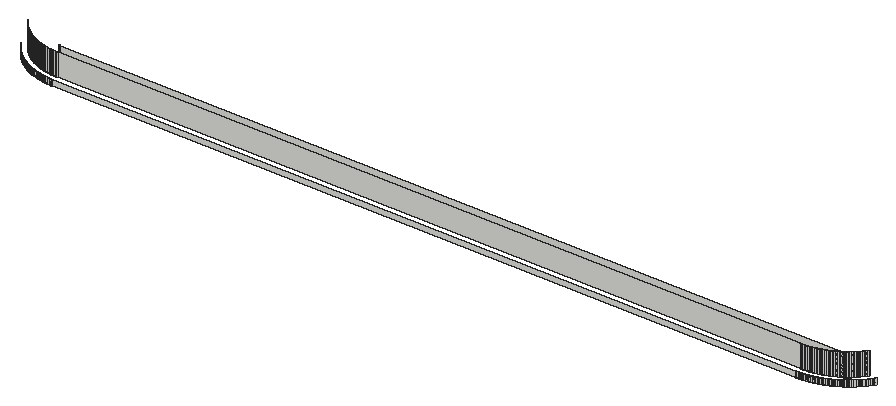
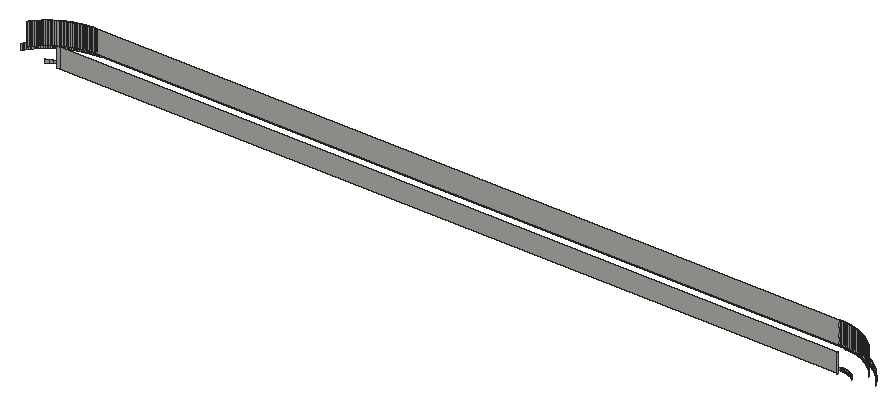
# SketchUp Ruby script. Lengths in inches.
U = 1.inch
M = Sketchup.active_model
def pt(a) = Geom::Point3d.new(a.map { |v| v * U })
def face(e, loops, mat)
  f = e.add_face(loops[0].map { |a| pt(a) })
  loops[1..].each { |l| e.add_face(l.map { |a| pt(a) }).erase! }
  f.material = f.back_material = mat if mat
  f
end
# faces: each face lists its corners as indices into pts; further lists are holes
def faces(e, pts, list, mat = nil) = list.each { |f| face(e, (f[0].is_a?(Array) ? f : [f]).map { |l| l.map { |i| pts[i] } }, mat) }
# xy, xz, yz: faces in a plane at the given z, y or x. An outline is a flat list of corners, or four numbers for a rectangle; further outlines are holes
def ring(l) = l.size == 4 ? [[l[0], l[1]], [l[2], l[1]], [l[2], l[3]], [l[0], l[3]]] : l.each_slice(2).to_a
def flat(e, list, mat, &to3) = list.each { |f| face(e, (f[0].is_a?(Array) ? f : [f]).map { |l| ring(l).map { |u, v| to3.(u, v) } }, mat) }
def xy(e, z, list, mat = nil) = flat(e, list, mat) { |x, y| [x, y, z] }
def xz(e, y, list, mat = nil) = flat(e, list, mat) { |x, z| [x, y, z] }
def yz(e, x, list, mat = nil) = flat(e, list, mat) { |y, z| [x, y, z] }
def lines(e, pts, list) = list.each { |a, b| e.add_line(pt(pts[a]), pt(pts[b])) }
# prism: a flat outline (further loops are holes) pulled along v
def prism(e, loops, v, mat = nil)
  f = face(e, loops, mat); d = Geom::Vector3d.new(v.map { |x| x * U })
  f.pushpull(f.normal.samedirection?(d) ? d.length : -d.length)
end
def box(e, o, s, mat = nil) = prism(e, [[o, [o[0] + s[0], o[1], o[2]], [o[0] + s[0], o[1] + s[1], o[2]], [o[0], o[1] + s[1], o[2]]]], [0, 0, s[2]], mat)
def at(x, y, z, deg = 0) = Geom::Transformation.translation(pt([x, y, z])) * Geom::Transformation.rotation(ORIGIN, Z_AXIS, deg.degrees)
def axes(o, x, y, z) = Geom::Transformation.new([*x, 0, *y, 0, *z, 0, *pt(o).to_a, 1])
def part(name) = M.definitions.add(name)
# library, detail: a bought-in or finely detailed component or shape, given as its bounding box
def library(name, o, s) = part(name).tap { |d| box(d.entities, o, s) }
def detail(e, o, s) = box(e.add_group.entities, o, s)
def put(e, d, t, mat = nil) = e.add_instance(d, t).tap { |i| i.material = mat if mat }
def group(e, t, mat = nil) = e.add_group.tap { |g| g.transformation = t; g.material = mat if mat }.entities
root = M.entities
xz(root,144,[[23.87,120,24.1875,122],[24.1875,120,290.26,122],[290.26,120,290.58,122]])
xz(root,146,[[23.9,122,24.1875,130],[24.1875,122,290.26,130],[290.26,122,290.55,130]])
xz(root,153,[[17.82,119,18,120],[18,119,296.45,120]])
xz(root,155,[[17.86,119,18,126],[18,119,296.45,126]])
xz(root,155.01,[[17.59,119,17.73,126]])
p = [[17.12,153.04,120],[16.94,153.0625,120],[16.94,153.0625,119],[17.12,153.04,119],[17.29,153.03,120],[17.29,153.03,119],
  [17.47,153.02,120],[17.47,153.02,119],[17.65,153.01,120],[17.65,153.01,119],[17.82,153,120],[17.82,153,119],
  [297.63,153.08,120],[296.45,153,120],[296.45,153,119],[297.63,153.08,119],[16.42,153.14,120],[16.24,153.17,120],
  [16.24,153.17,119],[16.42,153.14,119],[16.59,153.11,120],[16.59,153.11,119],[16.77,153.08,120],[16.77,153.08,119],
  [298.78,153.31,120],[298.78,153.31,119],[15.9,153.25,120],[15.73,153.29,120],[15.73,153.29,119],[15.9,153.25,119],
  [16.07,153.21,120],[16.07,153.21,119],[15.56,153.34,120],[15.39,153.39,120],[15.39,153.39,119],[15.56,153.34,119],
  [299.9,153.69,120],[299.9,153.69,119],[15.22,153.44,120],[15.05,153.5,120],[15.05,153.5,119],[15.22,153.44,119],
  [14.88,153.56,120],[14.88,153.56,119],[14.72,153.62,120],[14.56,153.69,120],[14.56,153.69,119],[14.72,153.62,119],
  [14.39,153.75,120],[14.39,153.75,119],[300.95,154.21,120],[300.95,154.21,119],[14.23,153.83,120],[14.07,153.9,120],
  [14.07,153.9,119],[14.23,153.83,119],[13.91,153.98,120],[13.91,153.98,119],[13.76,154.0625,120],[13.76,154.0625,119],
  [13.6,154.15,120],[13.45,154.24,120],[13.45,154.24,119],[13.6,154.15,119],[13.3,154.33,120],[13.3,154.33,119],
  [301.93,154.86,120],[301.93,154.86,119],[13.15,154.42,120],[13.15,154.42,119],[13,154.52,120],[13,154.52,119],
  [12.85,154.62,120],[12.85,154.62,119],[12.71,154.72,120],[12.71,154.72,119],[12.57,154.82,120],[12.57,154.82,119],
  [12.43,154.93,120],[12.43,154.93,119],[12.29,155.04,120],[12.29,155.04,119],[17.3125,155.03,126],[17.45,155.02,126],
  [17.45,155.02,119],[17.3125,155.03,119],[17.59,155.01,126],[17.59,155.01,119],[17.73,155.01,126],[17.86,155,126],
  [17.86,155,119],[17.73,155.01,119],[296.45,155,126],[297.37,155.06,126],[297.37,155.06,119],[296.45,155,119],
  [22.61,144.05,120],[22.92,144.03,120],[22.92,144.03,122],[22.61,144.05,122],[23.24,144.02,120],[23.24,144.02,122],
  [23.56,144.01,120],[23.56,144.01,122],[23.87,144,120],[23.87,144,122],[290.58,144,120],[290.9,144.01,120],
  [290.9,144.01,122],[290.58,144,122],[291.21,144.02,120],[291.21,144.02,122],[291.53,144.03,120],[291.53,144.03,122],
  [291.85,144.05,120],[291.85,144.05,122],[21.35,144.17,120],[21.66,144.13,120],[21.66,144.13,122],[21.35,144.17,122],
  [21.98,144.1,120],[21.98,144.1,122],[22.29,144.07,120],[22.29,144.07,122],[292.16,144.07,120],[292.16,144.07,122],
  [292.48,144.1,120],[292.48,144.1,122],[292.79,144.13,120],[292.79,144.13,122],[293.11,144.17,120],[293.11,144.17,122],
  [20.4,144.3,120],[20.72,144.25,120],[20.72,144.25,122],[20.4,144.3,122],[21.03,144.21,120],[21.03,144.21,122],
  [293.42,144.21,120],[293.42,144.21,122],[293.74,144.25,120],[293.74,144.25,122],[294.05,144.3,120],[294.05,144.3,122],
  [19.78,144.4,120],[20.09,144.35,120],[20.09,144.35,122],[19.78,144.4,122],[294.36,144.35,120],[294.36,144.35,122],
  [294.67,144.4,120],[294.67,144.4,122],[19.47,144.46,120],[19.47,144.46,122],[294.98,144.46,120],[294.98,144.46,122],
  [18.85,144.59,120],[19.16,144.52,120],[19.16,144.52,122],[18.85,144.59,122],[295.29,144.52,120],[295.29,144.52,122],
  [295.6,144.59,120],[295.6,144.59,122],[18.54,144.66,120],[18.54,144.66,122],[295.91,144.66,120],[295.91,144.66,122],
  [17.93,144.82,120],[18.23,144.74,120],[18.23,144.74,122],[17.93,144.82,122],[296.22,144.74,120],[296.22,144.74,122],
  [296.53,144.82,120],[296.53,144.82,122],[17.62,144.9,120],[17.62,144.9,122],[296.83,144.9,120],[296.83,144.9,122],
  [17.32,144.99,120],[17.32,144.99,122],[297.13,144.99,120],[297.13,144.99,122],[17.02,145.08,120],[17.02,145.08,122],
  [297.4375,145.08,120],[297.4375,145.08,122],[16.71,145.17,120],[16.71,145.17,122],[297.74,145.17,120],[297.74,145.17,122],
  [16.41,145.27,120],[16.41,145.27,122],[298.04,145.27,120],[298.04,145.27,122],[16.11,145.375,120],[16.11,145.375,122],
  [298.34,145.375,120],[298.34,145.375,122],[15.82,145.48,120],[15.82,145.48,122],[298.64,145.48,120],[298.64,145.48,122],
  [15.52,145.59,120],[15.52,145.59,122],[298.93,145.59,120],[298.93,145.59,122],[15.23,145.71,120],[15.23,145.71,122],
  [299.23,145.71,120],[299.23,145.71,122],[14.93,145.83,120],[14.93,145.83,122],[299.52,145.83,120],[299.52,145.83,122],
  [14.64,145.95,120],[14.64,145.95,122],[299.8125,145.95,120],[299.8125,145.95,122],[14.35,146.07,120],[14.35,146.07,122],
  [300.1,146.07,120],[300.1,146.07,122],[14.0625,146.2,120],[14.0625,146.2,122],[300.39,146.2,120],[300.39,146.2,122],
  [13.78,146.34,120],[13.78,146.34,122],[300.68,146.34,120],[300.68,146.34,122],[13.49,146.48,120],[13.49,146.48,122],
  [300.96,146.48,120],[300.96,146.48,122],[13.21,146.62,120],[13.21,146.62,122],[301.25,146.62,120],[301.25,146.62,122],
  [12.93,146.76,120],[12.93,146.76,122],[301.53,146.76,120],[301.53,146.76,122],[12.65,146.91,120],[12.65,146.91,122],
  [301.81,146.91,120],[301.81,146.91,122],[12.37,147.06,120],[12.37,147.06,122],[302.08,147.06,120],[302.08,147.06,122],
  [12.09,147.22,120],[12.09,147.22,122],[302.36,147.22,120],[302.36,147.22,122],[11.82,147.375,120],[11.82,147.375,122],
  [302.63,147.375,120],[302.63,147.375,122],[11.55,147.54,120],[11.55,147.54,122],[302.9,147.54,120],[302.9,147.54,122],
  [11.28,147.7,120],[11.28,147.7,122],[303.17,147.7,120],[303.17,147.7,122],[11.01,147.87,120],[11.01,147.87,122],
  [303.4375,147.87,120],[303.4375,147.87,122],[10.75,148.04,120],[10.75,148.04,122],[303.7,148.04,120],[303.7,148.04,122],
  [10.49,148.22,120],[10.49,148.22,122],[303.97,148.22,120],[303.97,148.22,122],[10.23,148.4,120],[10.23,148.4,122],
  [304.23,148.4,120],[304.23,148.4,122],[9.97,148.58,120],[9.97,148.58,122],[304.48,148.58,120],[304.48,148.58,122],
  [9.72,148.77,120],[9.72,148.77,122],[304.74,148.77,120],[304.74,148.77,122],[9.46,148.96,120],[9.46,148.96,122],
  [304.99,148.96,120],[304.99,148.96,122],[9.21,149.15,120],[9.21,149.15,122],[305.24,149.15,120],[305.24,149.15,122],
  [8.97,149.35,120],[8.97,149.35,122],[305.49,149.35,120],[305.49,149.35,122],[8.72,149.55,120],[8.72,149.55,122],
  [305.73,149.55,120],[305.73,149.55,122],[8.48,149.75,120],[8.48,149.75,122],[305.97,149.75,120],[305.97,149.75,122],
  [8.24,149.96,120],[8.24,149.96,122],[306.21,149.96,120],[306.21,149.96,122],[8,150.16,120],[8,150.16,122],
  [306.45,150.16,120],[306.45,150.16,122],[7.77,150.375,120],[7.77,150.375,122],[306.68,150.375,120],[306.68,150.375,122],
  [7.54,150.59,120],[7.54,150.59,122],[306.92,150.59,120],[306.92,150.59,122],[7.31,150.81,120],[7.31,150.81,122],
  [307.14,150.81,120],[307.14,150.81,122],[7.08,151.03,120],[7.08,151.03,122],[307.37,151.03,120],[307.37,151.03,122],
  [6.86,151.25,120],[6.86,151.25,122],[307.59,151.25,120],[307.59,151.25,122],[6.64,151.48,120],[6.64,151.48,122],
  [307.8125,151.48,120],[307.8125,151.48,122],[6.43,151.71,120],[6.43,151.71,122],[308.03,151.71,120],[308.03,151.71,122],
  [6.21,151.94,120],[6.21,151.94,122],[308.24,151.94,120],[308.24,151.94,122],[6,152.18,120],[6,152.18,122],
  [308.45,152.18,120],[308.45,152.18,122],[5.8,152.41,120],[5.8,152.41,122],[308.66,152.41,120],[308.66,152.41,122],
  [5.59,152.65,120],[5.59,152.65,122],[308.86,152.65,120],[308.86,152.65,122],[5.39,152.9,120],[5.39,152.9,122],
  [309.0625,152.9,120],[309.0625,152.9,122],[5.19,153.14,120],[5.19,153.14,122],[309.26,153.14,120],[309.26,153.14,122],
  [5,153.39,120],[5,153.39,122],[309.45,153.39,120],[309.45,153.39,122],[4.81,153.64,120],[4.81,153.64,122],
  [309.65,153.64,120],[309.65,153.64,122],[4.62,153.89,120],[4.62,153.89,122],[309.83,153.89,120],[309.83,153.89,122],
  [4.44,154.15,120],[4.44,154.15,122],[310.02,154.15,120],[310.02,154.15,122],[4.25,154.41,120],[4.25,154.41,122],
  [310.2,154.41,120],[310.2,154.41,122],[4.08,154.67,120],[4.08,154.67,122],[310.375,154.67,120],[310.375,154.67,122],
  [3.9,154.93,120],[3.9,154.93,122],[310.55,154.93,120],[310.55,154.93,122],[22.45,146.07,122],[22.74,146.05,122],
  [22.74,146.05,130],[22.45,146.07,130],[23.03,146.03,122],[23.03,146.03,130],[23.32,146.02,122],[23.32,146.02,130],
  [23.61,146.01,122],[23.61,146.01,130],[23.9,146,122],[23.9,146,130],[290.55,146,122],[290.85,146.01,122],
  [290.85,146.01,130],[290.55,146,130],[291.14,146.02,122],[291.14,146.02,130],[291.43,146.03,122],[291.43,146.03,130],
  [291.71,146.05,122],[291.71,146.05,130],[292,146.07,122],[292,146.07,130],[21.58,146.15,122],[21.87,146.12,122],
  [21.87,146.12,130],[21.58,146.15,130],[22.16,146.09,122],[22.16,146.09,130],[292.29,146.09,122],[292.29,146.09,130],
  [292.58,146.12,122],[292.58,146.12,130],[292.87,146.15,122],[292.87,146.15,130],[20.72,146.27,122],[21.01,146.23,122],
  [21.01,146.23,130],[20.72,146.27,130],[21.29,146.1875,122],[21.29,146.1875,130],[293.16,146.1875,122],[293.16,146.1875,130],
  [293.45,146.23,122],[293.45,146.23,130],[293.73,146.27,122],[293.73,146.27,130],[20.15,146.37,122],[20.43,146.32,122],
  [20.43,146.32,130],[20.15,146.37,130],[294.02,146.32,122],[294.02,146.32,130],[294.31,146.37,122],[294.31,146.37,130],
  [19.58,146.48,122],[19.86,146.42,122],[19.86,146.42,130],[19.58,146.48,130],[294.59,146.42,122],[294.59,146.42,130],
  [294.875,146.48,122],[294.875,146.48,130],[19.01,146.61,122],[19.3,146.54,122],[19.3,146.54,130],[19.01,146.61,130],
  [295.16,146.54,122],[295.16,146.54,130],[295.44,146.61,122],[295.44,146.61,130],[18.73,146.68,122],[18.73,146.68,130],
  [295.72,146.68,122],[295.72,146.68,130],[18.17,146.83,122],[18.45,146.75,122],[18.45,146.75,130],[18.17,146.83,130],
  [296,146.75,122],[296,146.75,130],[296.28,146.83,122],[296.28,146.83,130],[17.89,146.91,122],[17.89,146.91,130],
  [296.5625,146.91,122],[296.5625,146.91,130],[17.61,146.99,122],[17.61,146.99,130],[296.84,146.99,122],[296.84,146.99,130],
  [17.34,147.08,122],[17.34,147.08,130],[297.12,147.08,122],[297.12,147.08,130],[17.0625,147.17,122],[17.0625,147.17,130],
  [297.39,147.17,122],[297.39,147.17,130],[16.79,147.26,122],[16.79,147.26,130],[297.67,147.26,122],[297.67,147.26,130],
  [16.51,147.36,122],[16.51,147.36,130],[297.9375,147.36,122],[297.9375,147.36,130],[16.24,147.46,122],[16.24,147.46,130],
  [298.21,147.46,122],[298.21,147.46,130],[15.97,147.57,122],[15.97,147.57,130],[298.48,147.57,122],[298.48,147.57,130],
  [15.7,147.67,122],[15.7,147.67,130],[298.75,147.67,122],[298.75,147.67,130],[15.4375,147.79,122],[15.4375,147.79,130],
  [299.02,147.79,122],[299.02,147.79,130],[15.17,147.9,122],[15.17,147.9,130],[299.28,147.9,122],[299.28,147.9,130],
  [14.91,148.02,122],[14.91,148.02,130],[299.55,148.02,122],[299.55,148.02,130],[14.64,148.14,122],[14.64,148.14,130],
  [299.81,148.14,122],[299.81,148.14,130],[14.38,148.27,122],[14.38,148.27,130],[300.07,148.27,122],[300.07,148.27,130],
  [14.12,148.4,122],[14.12,148.4,130],[300.33,148.4,122],[300.33,148.4,130],[13.86,148.53,122],[13.86,148.53,130],
  [300.59,148.53,122],[300.59,148.53,130],[13.61,148.67,122],[13.61,148.67,130],[300.84,148.67,122],[300.84,148.67,130],
  [13.35,148.81,122],[13.35,148.81,130],[301.1,148.81,122],[301.1,148.81,130],[13.1,148.95,122],[13.1,148.95,130],
  [301.35,148.95,122],[301.35,148.95,130],[12.85,149.09,122],[12.85,149.09,130],[301.6,149.09,122],[301.6,149.09,130],
  [12.6,149.24,122],[12.6,149.24,130],[301.85,149.24,122],[301.85,149.24,130],[12.36,149.39,122],[12.36,149.39,130],
  [302.1,149.39,122],[302.1,149.39,130],[12.11,149.55,122],[12.11,149.55,130],[302.34,149.55,122],[302.34,149.55,130],
  [11.87,149.71,122],[11.87,149.71,130],[302.58,149.71,122],[302.58,149.71,130],[11.63,149.87,122],[11.63,149.87,130],
  [302.82,149.87,122],[302.82,149.87,130],[11.39,150.03,122],[11.39,150.03,130],[303.0625,150.03,122],[303.0625,150.03,130],
  [11.16,150.2,122],[11.16,150.2,130],[303.3,150.2,122],[303.3,150.2,130],[10.92,150.37,122],[10.92,150.37,130],
  [303.53,150.37,122],[303.53,150.37,130],[10.69,150.55,122],[10.69,150.55,130],[303.76,150.55,122],[303.76,150.55,130],
  [10.46,150.72,122],[10.46,150.72,130],[303.99,150.72,122],[303.99,150.72,130],[10.23,150.9,122],[10.23,150.9,130],
  [304.22,150.9,122],[304.22,150.9,130],[10.01,151.09,122],[10.01,151.09,130],[304.44,151.09,122],[304.44,151.09,130],
  [9.79,151.27,122],[9.79,151.27,130],[304.66,151.27,122],[304.66,151.27,130],[9.57,151.46,122],[9.57,151.46,130],
  [304.88,151.46,122],[304.88,151.46,130],[9.35,151.65,122],[9.35,151.65,130],[305.1,151.65,122],[305.1,151.65,130],
  [9.14,151.84,122],[9.14,151.84,130],[305.32,151.84,122],[305.32,151.84,130],[8.93,152.04,122],[8.93,152.04,130],
  [305.53,152.04,122],[305.53,152.04,130],[8.72,152.24,122],[8.72,152.24,130],[305.74,152.24,122],[305.74,152.24,130],
  [8.51,152.44,122],[8.51,152.44,130],[305.94,152.44,122],[305.94,152.44,130],[8.31,152.65,122],[8.31,152.65,130],
  [306.15,152.65,122],[306.15,152.65,130],[8.11,152.86,122],[8.11,152.86,130],[306.35,152.86,122],[306.35,152.86,130],
  [7.91,153.07,122],[7.91,153.07,130],[306.55,153.07,122],[306.55,153.07,130],[7.71,153.28,122],[7.71,153.28,130],
  [306.74,153.28,122],[306.74,153.28,130],[7.52,153.49,122],[7.52,153.49,130],[306.94,153.49,122],[306.94,153.49,130],
  [7.33,153.71,122],[7.33,153.71,130],[307.125,153.71,122],[307.125,153.71,130],[7.14,153.93,122],[7.14,153.93,130],
  [307.3125,153.93,122],[307.3125,153.93,130],[6.96,154.15,122],[6.96,154.15,130],[307.5,154.15,122],[307.5,154.15,130],
  [6.78,154.38,122],[6.78,154.38,130],[307.68,154.38,122],[307.68,154.38,130],[6.6,154.61,122],[6.6,154.61,130],
  [307.86,154.61,122],[307.86,154.61,130],[6.42,154.84,122],[6.42,154.84,130],[308.03,154.84,122],[308.03,154.84,130],
  [6.25,155.07,122],[6.25,155.07,130],[308.2,155.07,122],[308.2,155.07,130]]
faces(root,p,[[0,1,2,3],[4,0,3,5],[6,4,5,7],[8,6,7,9],[10,8,9,11],[12,13,14,15],[16,17,18,19],[20,16,19,21],
  [22,20,21,23],[1,22,23,2],[24,12,15,25],[26,27,28,29],[30,26,29,31],[17,30,31,18],[32,33,34,35],[27,32,35,28],
  [36,24,25,37],[38,39,40,41],[33,38,41,34],[39,42,43,40],[44,45,46,47],[42,44,47,43],[45,48,49,46],[50,36,37,51],
  [52,53,54,55],[48,52,55,49],[53,56,57,54],[56,58,59,57],[60,61,62,63],[58,60,63,59],[61,64,65,62],[66,50,51,67],
  [64,68,69,65],[68,70,71,69],[70,72,73,71],[72,74,75,73],[74,76,77,75],[76,78,79,77],[78,80,81,79],[82,83,84,85],
  [83,86,87,84],[88,89,90,91],[92,93,94,95],[96,97,98,99],[97,100,101,98],[100,102,103,101],[102,104,105,103],[106,107,108,109],
  [107,110,111,108],[110,112,113,111],[112,114,115,113],[116,117,118,119],[117,120,121,118],[120,122,123,121],[122,96,99,123],[114,124,125,115],
  [124,126,127,125],[126,128,129,127],[128,130,131,129],[132,133,134,135],[133,136,137,134],[136,116,119,137],[130,138,139,131],[138,140,141,139],
  [140,142,143,141],[144,145,146,147],[145,132,135,146],[142,148,149,143],[148,150,151,149],[152,144,147,153],[150,154,155,151],[156,157,158,159],
  [157,152,153,158],[154,160,161,155],[160,162,163,161],[164,156,159,165],[162,166,167,163],[168,169,170,171],[169,164,165,170],[166,172,173,167],
  [172,174,175,173],[176,168,171,177],[174,178,179,175],[180,176,177,181],[178,182,183,179],[184,180,181,185],[182,186,187,183],[188,184,185,189],
  [186,190,191,187],[192,188,189,193],[190,194,195,191],[196,192,193,197],[194,198,199,195],[200,196,197,201],[198,202,203,199],[204,200,201,205],
  [202,206,207,203],[208,204,205,209],[206,210,211,207],[212,208,209,213],[210,214,215,211],[216,212,213,217],[214,218,219,215],[220,216,217,221],
  [218,222,223,219],[224,220,221,225],[222,226,227,223],[228,224,225,229],[226,230,231,227],[232,228,229,233],[230,234,235,231],[236,232,233,237],
  [234,238,239,235],[240,236,237,241],[238,242,243,239],[244,240,241,245],[242,246,247,243],[248,244,245,249],[246,250,251,247],[252,248,249,253],
  [250,254,255,251],[256,252,253,257],[254,258,259,255],[260,256,257,261],[258,262,263,259],[264,260,261,265],[262,266,267,263],[268,264,265,269],
  [266,270,271,267],[272,268,269,273],[270,274,275,271],[276,272,273,277],[274,278,279,275],[280,276,277,281],[278,282,283,279],[284,280,281,285],
  [282,286,287,283],[288,284,285,289],[286,290,291,287],[292,288,289,293],[290,294,295,291],[296,292,293,297],[294,298,299,295],[300,296,297,301],
  [298,302,303,299],[304,300,301,305],[302,306,307,303],[308,304,305,309],[306,310,311,307],[312,308,309,313],[310,314,315,311],[316,312,313,317],
  [314,318,319,315],[320,316,317,321],[318,322,323,319],[324,320,321,325],[322,326,327,323],[328,324,325,329],[326,330,331,327],[332,328,329,333],
  [330,334,335,331],[336,332,333,337],[334,338,339,335],[340,336,337,341],[338,342,343,339],[344,340,341,345],[342,346,347,343],[348,344,345,349],
  [346,350,351,347],[352,348,349,353],[350,354,355,351],[356,352,353,357],[354,358,359,355],[360,356,357,361],[358,362,363,359],[364,360,361,365],
  [362,366,367,363],[368,364,365,369],[366,370,371,367],[372,368,369,373],[370,374,375,371],[376,372,373,377],[374,378,379,375],[380,376,377,381],
  [378,382,383,379],[384,380,381,385],[382,386,387,383],[388,384,385,389],[386,390,391,387],[392,388,389,393],[390,394,395,391],[396,392,393,397],
  [394,398,399,395],[400,401,402,403],[401,404,405,402],[404,406,407,405],[406,408,409,407],[408,410,411,409],[412,413,414,415],[413,416,417,414],
  [416,418,419,417],[418,420,421,419],[420,422,423,421],[424,425,426,427],[425,428,429,426],[428,400,403,429],[422,430,431,423],[430,432,433,431],
  [432,434,435,433],[436,437,438,439],[437,440,441,438],[440,424,427,441],[434,442,443,435],[442,444,445,443],[444,446,447,445],[448,449,450,451],
  [449,436,439,450],[446,452,453,447],[452,454,455,453],[456,457,458,459],[457,448,451,458],[454,460,461,455],[460,462,463,461],[464,465,466,467],
  [465,456,459,466],[462,468,469,463],[468,470,471,469],[472,464,467,473],[470,474,475,471],[476,477,478,479],[477,472,473,478],[474,480,481,475],
  [480,482,483,481],[484,476,479,485],[482,486,487,483],[488,484,485,489],[486,490,491,487],[492,488,489,493],[490,494,495,491],[496,492,493,497],
  [494,498,499,495],[500,496,497,501],[498,502,503,499],[504,500,501,505],[502,506,507,503],[508,504,505,509],[506,510,511,507],[512,508,509,513],
  [510,514,515,511],[516,512,513,517],[514,518,519,515],[520,516,517,521],[518,522,523,519],[524,520,521,525],[522,526,527,523],[528,524,525,529],
  [526,530,531,527],[532,528,529,533],[530,534,535,531],[536,532,533,537],[534,538,539,535],[540,536,537,541],[538,542,543,539],[544,540,541,545],
  [542,546,547,543],[548,544,545,549],[546,550,551,547],[552,548,549,553],[550,554,555,551],[556,552,553,557],[554,558,559,555],[560,556,557,561],
  [558,562,563,559],[564,560,561,565],[562,566,567,563],[568,564,565,569],[566,570,571,567],[572,568,569,573],[570,574,575,571],[576,572,573,577],
  [574,578,579,575],[580,576,577,581],[578,582,583,579],[584,580,581,585],[582,586,587,583],[588,584,585,589],[586,590,591,587],[592,588,589,593],
  [590,594,595,591],[596,592,593,597],[594,598,599,595],[600,596,597,601],[598,602,603,599],[604,600,601,605],[602,606,607,603],[608,604,605,609],
  [606,610,611,607],[612,608,609,613],[610,614,615,611],[616,612,613,617],[614,618,619,615],[620,616,617,621],[618,622,623,619],[624,620,621,625],
  [622,626,627,623],[628,624,625,629],[626,630,631,627],[632,628,629,633],[630,634,635,631],[636,632,633,637],[634,638,639,635],[640,636,637,641],
  [638,642,643,639],[644,640,641,645],[642,646,647,643],[648,644,645,649],[646,650,651,647],[652,648,649,653],[650,654,655,651],[656,652,653,657],
  [654,658,659,655],[660,656,657,661],[658,662,663,659],[664,660,661,665],[662,666,667,663],[668,664,665,669],[666,670,671,667],[672,668,669,673],
  [670,674,675,671],[676,672,673,677],[674,678,679,675],[680,676,677,681],[678,682,683,679],[684,680,681,685],[682,686,687,683]])
